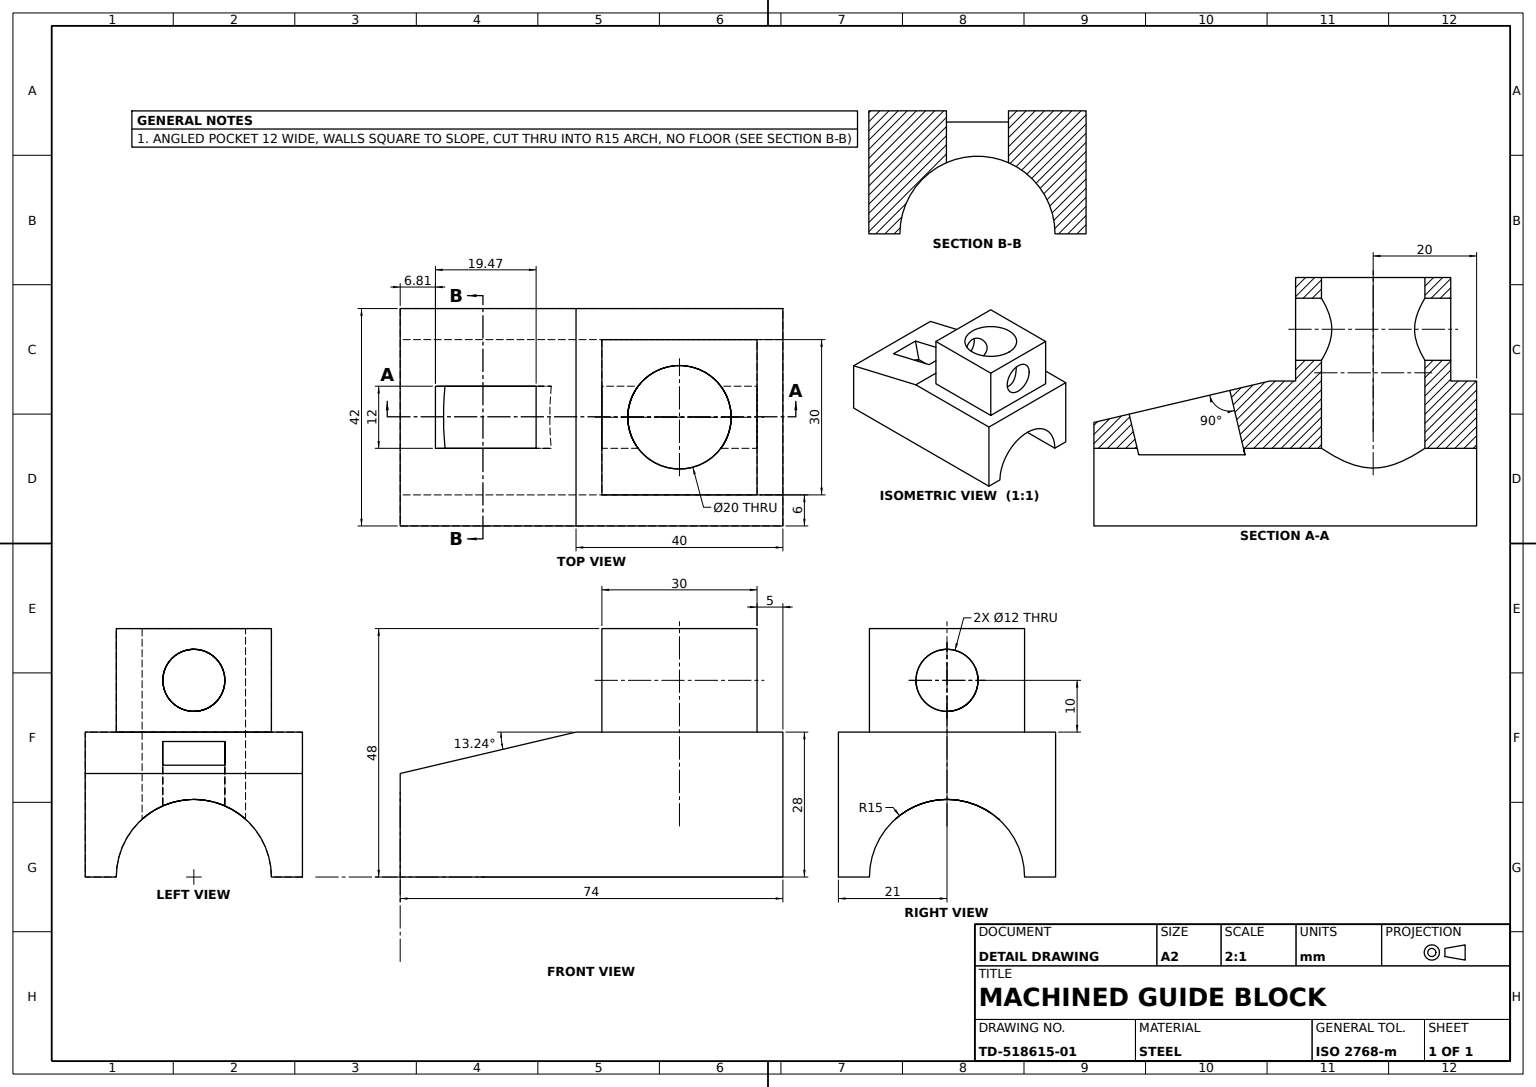
ISO-10303-21;
HEADER;
FILE_DESCRIPTION((''),'2;1');
FILE_NAME('','',(''),(''),'','','');
FILE_SCHEMA(('AUTOMOTIVE_DESIGN'));
ENDSEC;
DATA;
#1=APPLICATION_CONTEXT('');
#2=PRODUCT_CONTEXT('',#1,'mechanical');
#3=PRODUCT('','','',(#2));
#4=PRODUCT_DEFINITION_FORMATION('','',#3);
#5=PRODUCT_DEFINITION_CONTEXT('',#1,'design');
#6=PRODUCT_DEFINITION('','',#4,#5);
#7=PRODUCT_DEFINITION_SHAPE('','',#6);
#8=(LENGTH_UNIT()NAMED_UNIT(*)SI_UNIT(.MILLI.,.METRE.));
#9=(NAMED_UNIT(*)PLANE_ANGLE_UNIT()SI_UNIT($,.RADIAN.));
#10=(NAMED_UNIT(*)SI_UNIT($,.STERADIAN.)SOLID_ANGLE_UNIT());
#11=UNCERTAINTY_MEASURE_WITH_UNIT(LENGTH_MEASURE(1.E-05),#8,'distance_accuracy_value','');
#12=(GEOMETRIC_REPRESENTATION_CONTEXT(3)GLOBAL_UNCERTAINTY_ASSIGNED_CONTEXT((#11))GLOBAL_UNIT_ASSIGNED_CONTEXT((#8,#9,#10))REPRESENTATION_CONTEXT('',''));
#13=CARTESIAN_POINT('',(69.,28.,6.));
#14=VERTEX_POINT('',#13);
#15=CARTESIAN_POINT('',(39.,28.,6.));
#16=VERTEX_POINT('',#15);
#17=DIRECTION('',(-1.,0.,0.));
#18=VECTOR('',#17,1000.);
#19=LINE('',#15,#18);
#20=EDGE_CURVE('',#14,#16,#19,.T.);
#21=ORIENTED_EDGE('',*,*,#20,.T.);
#22=CARTESIAN_POINT('',(39.,48.,6.));
#23=VERTEX_POINT('',#22);
#24=DIRECTION('',(0.,-1.,0.));
#25=VECTOR('',#24,1000.);
#26=LINE('',#22,#25);
#27=EDGE_CURVE('',#23,#16,#26,.T.);
#28=ORIENTED_EDGE('',*,*,#27,.F.);
#29=CARTESIAN_POINT('',(69.,48.,6.));
#30=VERTEX_POINT('',#29);
#31=LINE('',#22,#18);
#32=EDGE_CURVE('',#30,#23,#31,.T.);
#33=ORIENTED_EDGE('',*,*,#32,.F.);
#34=LINE('',#29,#25);
#35=EDGE_CURVE('',#30,#14,#34,.T.);
#36=ORIENTED_EDGE('',*,*,#35,.T.);
#37=EDGE_LOOP('',(#21,#28,#33,#36));
#38=FACE_OUTER_BOUND('',#37,.T.);
#39=DIRECTION('',(0.,0.,1.));
#40=DIRECTION('',(1.,0.,0.));
#41=AXIS2_PLACEMENT_3D('',#22,#39,#40);
#42=PLANE('',#41);
#43=ADVANCED_FACE('',(#38),#42,.F.);
#44=CARTESIAN_POINT('',(8.662284,13.747727,27.));
#45=VERTEX_POINT('',#44);
#46=CARTESIAN_POINT('',(6.81392,21.603275,27.));
#47=VERTEX_POINT('',#46);
#48=CARTESIAN_POINT('',(15.154904,-13.845905,27.));
#49=DIRECTION('',(-0.229039334,0.973417168,0.));
#50=VECTOR('',#49,1000.);
#51=LINE('',#48,#50);
#52=EDGE_CURVE('',#45,#47,#51,.T.);
#53=ORIENTED_EDGE('',*,*,#52,.F.);
#54=CARTESIAN_POINT('',(8.662284,13.747727,15.));
#55=VERTEX_POINT('',#54);
#56=CARTESIAN_POINT('',(8.263626,15.442026,23.117874));
#57=CARTESIAN_POINT('',(8.263626,15.442026,18.882126));
#58=(BOUNDED_CURVE()B_SPLINE_CURVE(3,(#44,#56,#57,#54),.UNSPECIFIED.,.F.,.F.)B_SPLINE_CURVE_WITH_KNOTS((4,4),(5.871668461,6.694702153),.UNSPECIFIED.)CURVE()GEOMETRIC_REPRESENTATION_ITEM()RATIONAL_B_SPLINE_CURVE((1.,0.944343426,0.944343426,1.))REPRESENTATION_ITEM(''));
#59=EDGE_CURVE('',#45,#55,#58,.T.);
#60=ORIENTED_EDGE('',*,*,#59,.T.);
#61=CARTESIAN_POINT('',(6.81392,21.603275,15.));
#62=VERTEX_POINT('',#61);
#63=CARTESIAN_POINT('',(15.154904,-13.845905,15.));
#64=LINE('',#63,#50);
#65=EDGE_CURVE('',#55,#62,#64,.T.);
#66=ORIENTED_EDGE('',*,*,#65,.T.);
#67=CARTESIAN_POINT('',(6.81392,21.603275,21.));
#68=VECTOR('',#39,1000.);
#69=LINE('',#67,#68);
#70=EDGE_CURVE('',#62,#47,#69,.T.);
#71=ORIENTED_EDGE('',*,*,#70,.T.);
#72=EDGE_LOOP('',(#53,#60,#66,#71));
#73=FACE_OUTER_BOUND('',#72,.T.);
#74=CARTESIAN_POINT('',(15.154904,-13.845905,21.));
#75=DIRECTION('',(-0.973417168,-0.229039334,0.));
#76=DIRECTION('',(0.229039334,-0.973417168,0.));
#77=AXIS2_PLACEMENT_3D('',#74,#75,#76);
#78=PLANE('',#77);
#79=ADVANCED_FACE('',(#73),#78,.F.);
#80=CARTESIAN_POINT('',(44.,15.,21.));
#81=VERTEX_POINT('',#80);
#82=CARTESIAN_POINT('',(64.,15.,21.));
#83=VERTEX_POINT('',#82);
#84=CARTESIAN_POINT('',(44.,15.,20.315766));
#85=CARTESIAN_POINT('',(44.069456,14.953444,19.646642));
#86=CARTESIAN_POINT('',(44.338112,14.776396,18.336319));
#87=CARTESIAN_POINT('',(44.540827,14.643657,17.690301));
#88=CARTESIAN_POINT('',(45.054072,14.317485,16.483317));
#89=CARTESIAN_POINT('',(45.365864,14.123132,15.913734));
#90=CARTESIAN_POINT('',(46.093085,13.690648,14.843775));
#91=CARTESIAN_POINT('',(46.499373,13.457922,14.35618));
#92=CARTESIAN_POINT('',(47.39588,12.979625,13.464394));
#93=CARTESIAN_POINT('',(47.891028,12.7318,13.057623));
#94=CARTESIAN_POINT('',(48.941558,12.262423,12.350546));
#95=CARTESIAN_POINT('',(49.498495,12.039444,12.047121));
#96=CARTESIAN_POINT('',(50.390776,11.745112,11.668446));
#97=CARTESIAN_POINT('',(50.699259,11.653393,11.554638));
#98=CARTESIAN_POINT('',(51.33166,11.490287,11.356882));
#99=CARTESIAN_POINT('',(51.65257,11.419613,11.27373));
#100=CARTESIAN_POINT('',(52.304444,11.303629,11.139176));
#101=CARTESIAN_POINT('',(52.635408,11.258325,11.087771));
#102=CARTESIAN_POINT('',(53.308259,11.196708,11.018222));
#103=CARTESIAN_POINT('',(53.652096,11.180607,11.000299));
#104=CARTESIAN_POINT('',(54.669733,11.179816,10.999414));
#105=CARTESIAN_POINT('',(55.33834,11.241429,11.067135));
#106=CARTESIAN_POINT('',(56.327525,11.415429,11.26882));
#107=CARTESIAN_POINT('',(56.651266,11.486374,11.352241));
#108=CARTESIAN_POINT('',(57.280293,11.647657,11.547586));
#109=CARTESIAN_POINT('',(57.586917,11.738226,11.659782));
#110=CARTESIAN_POINT('',(58.18588,11.934889,11.912423));
#111=CARTESIAN_POINT('',(58.479453,12.0415,12.053601));
#112=CARTESIAN_POINT('',(59.045381,12.263283,12.360111));
#113=CARTESIAN_POINT('',(59.318063,12.37846,12.525395));
#114=CARTESIAN_POINT('',(59.844751,12.613707,12.879679));
#115=CARTESIAN_POINT('',(60.098751,12.733786,13.068682));
#116=CARTESIAN_POINT('',(60.589028,12.97574,13.471037));
#117=CARTESIAN_POINT('',(60.826316,13.098175,13.685453));
#118=CARTESIAN_POINT('',(61.502941,13.459144,14.358416));
#119=CARTESIAN_POINT('',(61.907554,13.691086,14.845407));
#120=CARTESIAN_POINT('',(62.4469,14.011753,15.637912));
#121=CARTESIAN_POINT('',(62.615307,14.114119,15.912494));
#122=CARTESIAN_POINT('',(62.928321,14.307332,16.484325));
#123=CARTESIAN_POINT('',(63.07303,14.398263,16.782352));
#124=CARTESIAN_POINT('',(63.459729,14.644004,17.691343));
#125=CARTESIAN_POINT('',(63.65875,14.774335,18.323429));
#126=CARTESIAN_POINT('',(63.862792,14.908791,19.315004));
#127=CARTESIAN_POINT('',(63.914681,14.943234,19.653364));
#128=CARTESIAN_POINT('',(63.982998,14.988649,20.326153));
#129=CARTESIAN_POINT('',(64.,15.,20.662901));
#130=B_SPLINE_CURVE_WITH_KNOTS('',3,(#80,#84,#85,#86,#87,#88,#89,#90,#91,#92,#93,#94,#95,#96,#97,#98,#99,#100,#101,#102,#103,#104,#105,#106,#107,#108,#109,#110,#111,#112,#113,#114,#115,#116,#117,#118,#119,#120,#121,#122,#123,#124,#125,#126,#127,#128,#129,#82),.UNSPECIFIED.,.F.,.F.,(4,2,2,2,2,2,2,2,2,2,2,2,2,2,2,2,2,2,2,2,2,2,2,4),(0.,0.002019983,0.004039966,0.006059949,0.008079932,0.010099915,0.012119898,0.013129889,0.014139881,0.015149872,0.016159864,0.018179847,0.019189838,0.02019983,0.021209821,0.022219812,0.023229804,0.024239795,0.026259778,0.02726977,0.028279761,0.030299744,0.031309736,0.032319727),.UNSPECIFIED.);
#131=EDGE_CURVE('',#81,#83,#130,.T.);
#132=ORIENTED_EDGE('',*,*,#131,.F.);
#133=CARTESIAN_POINT('',(64.,15.,21.336653));
#134=CARTESIAN_POINT('',(63.983044,14.98868,21.673657));
#135=CARTESIAN_POINT('',(63.914478,14.943099,22.348377));
#136=CARTESIAN_POINT('',(63.862521,14.908613,22.686291));
#137=CARTESIAN_POINT('',(63.659358,14.774736,23.673654));
#138=CARTESIAN_POINT('',(63.460738,14.64464,24.306492));
#139=CARTESIAN_POINT('',(63.071809,14.397489,25.220414));
#140=CARTESIAN_POINT('',(62.927942,14.3071,25.516335));
#141=CARTESIAN_POINT('',(62.616155,14.114641,26.085991));
#142=CARTESIAN_POINT('',(62.447797,14.012288,26.360755));
#143=CARTESIAN_POINT('',(61.90617,13.69026,27.156655));
#144=CARTESIAN_POINT('',(61.492918,13.4536,27.652569));
#145=CARTESIAN_POINT('',(60.594478,12.974694,28.544094));
#146=CARTESIAN_POINT('',(60.107726,12.731094,28.943623));
#147=CARTESIAN_POINT('',(59.31506,12.377155,29.476526));
#148=CARTESIAN_POINT('',(59.039253,12.260777,29.643428));
#149=CARTESIAN_POINT('',(58.474857,12.039806,29.948664));
#150=CARTESIAN_POINT('',(58.185318,11.934736,30.087761));
#151=CARTESIAN_POINT('',(57.590293,11.739303,30.338847));
#152=CARTESIAN_POINT('',(57.284813,11.648933,30.450844));
#153=CARTESIAN_POINT('',(56.655932,11.487455,30.646474));
#154=CARTESIAN_POINT('',(56.330246,11.416025,30.730479));
#155=CARTESIAN_POINT('',(55.345423,11.242442,30.931711));
#156=CARTESIAN_POINT('',(54.676284,11.179925,31.000464));
#157=CARTESIAN_POINT('',(53.651615,11.180551,30.999764));
#158=CARTESIAN_POINT('',(53.310132,11.196628,30.981866));
#159=CARTESIAN_POINT('',(52.639673,11.257844,30.912774));
#160=CARTESIAN_POINT('',(52.30873,11.302959,30.861593));
#161=CARTESIAN_POINT('',(51.654892,11.419108,30.726864));
#162=CARTESIAN_POINT('',(51.330007,11.490688,30.642637));
#163=CARTESIAN_POINT('',(50.698906,11.653509,30.445215));
#164=CARTESIAN_POINT('',(50.393107,11.7444,30.332447));
#165=CARTESIAN_POINT('',(49.501422,12.038365,29.954313));
#166=CARTESIAN_POINT('',(48.94037,12.262732,29.649261));
#167=CARTESIAN_POINT('',(47.8791,12.737353,28.933735));
#168=CARTESIAN_POINT('',(47.39227,12.98147,28.532433));
#169=CARTESIAN_POINT('',(46.720293,13.3401,27.863365));
#170=CARTESIAN_POINT('',(46.506134,13.458444,27.629057));
#171=CARTESIAN_POINT('',(46.09759,13.690134,27.136314));
#172=CARTESIAN_POINT('',(45.903795,13.803175,26.878281));
#173=CARTESIAN_POINT('',(45.364101,14.124275,26.082531));
#174=CARTESIAN_POINT('',(45.055173,14.316803,25.51853));
#175=CARTESIAN_POINT('',(44.671193,14.560799,24.616644));
#176=CARTESIAN_POINT('',(44.556546,14.634651,24.306638));
#177=CARTESIAN_POINT('',(44.356066,14.764811,23.665935));
#178=CARTESIAN_POINT('',(44.27196,14.819993,23.340409));
#179=CARTESIAN_POINT('',(44.069686,14.953289,22.355722));
#180=CARTESIAN_POINT('',(44.,15.,21.68333));
#181=B_SPLINE_CURVE_WITH_KNOTS('',3,(#82,#133,#134,#135,#136,#137,#138,#139,#140,#141,#142,#143,#144,#145,#146,#147,#148,#149,#150,#151,#152,#153,#154,#155,#156,#157,#158,#159,#160,#161,#162,#163,#164,#165,#166,#167,#168,#169,#170,#171,#172,#173,#174,#175,#176,#177,#178,#179,#180,#80),.UNSPECIFIED.,.F.,.F.,(4,2,2,2,2,2,2,2,2,2,2,2,2,2,2,2,2,2,2,2,2,2,2,2,4),(0.032319727,0.033328384,0.034337041,0.036354356,0.037363013,0.03837167,0.040388984,0.042406298,0.043414955,0.044423612,0.04543227,0.046440927,0.048458241,0.049466898,0.050475555,0.051484212,0.052492869,0.054510184,0.056527498,0.057536155,0.058544812,0.060562126,0.061570783,0.06257944,0.064596755),.UNSPECIFIED.);
#182=EDGE_CURVE('',#83,#81,#181,.T.);
#183=ORIENTED_EDGE('',*,*,#182,.F.);
#184=EDGE_LOOP('',(#132,#183));
#185=FACE_BOUND('',#184,.T.);
#186=CARTESIAN_POINT('',(0.,0.,6.));
#187=VERTEX_POINT('',#186);
#188=CARTESIAN_POINT('',(0.,0.,36.));
#189=VERTEX_POINT('',#188);
#190=CARTESIAN_POINT('',(0.,0.,21.));
#191=DIRECTION('',(0.,1.,0.));
#192=AXIS2_PLACEMENT_3D('',#190,#40,#191);
#193=CIRCLE('',#192,15.);
#194=EDGE_CURVE('',#187,#189,#193,.T.);
#195=ORIENTED_EDGE('',*,*,#194,.F.);
#196=CARTESIAN_POINT('',(74.,0.,6.));
#197=VERTEX_POINT('',#196);
#198=CARTESIAN_POINT('',(164.616747,0.,6.));
#199=LINE('',#198,#18);
#200=EDGE_CURVE('',#197,#187,#199,.T.);
#201=ORIENTED_EDGE('',*,*,#200,.F.);
#202=CARTESIAN_POINT('',(74.,0.,36.));
#203=VERTEX_POINT('',#202);
#204=CARTESIAN_POINT('',(74.,0.,21.));
#205=AXIS2_PLACEMENT_3D('',#204,#17,#39);
#206=CIRCLE('',#205,15.);
#207=EDGE_CURVE('',#203,#197,#206,.T.);
#208=ORIENTED_EDGE('',*,*,#207,.F.);
#209=CARTESIAN_POINT('',(164.616747,0.,36.));
#210=LINE('',#209,#18);
#211=EDGE_CURVE('',#203,#189,#210,.T.);
#212=ORIENTED_EDGE('',*,*,#211,.T.);
#213=EDGE_LOOP('',(#195,#201,#208,#212));
#214=FACE_OUTER_BOUND('',#213,.T.);
#215=CARTESIAN_POINT('',(29.20846,13.747727,15.));
#216=VERTEX_POINT('',#215);
#217=CARTESIAN_POINT('',(29.20846,13.747727,27.));
#218=VERTEX_POINT('',#217);
#219=CARTESIAN_POINT('',(28.809801,15.442026,18.882126));
#220=CARTESIAN_POINT('',(28.809801,15.442026,23.117874));
#221=(BOUNDED_CURVE()B_SPLINE_CURVE(3,(#215,#219,#220,#217),.UNSPECIFIED.,.F.,.F.)B_SPLINE_CURVE_WITH_KNOTS((4,4),(5.871668461,6.694702153),.UNSPECIFIED.)CURVE()GEOMETRIC_REPRESENTATION_ITEM()RATIONAL_B_SPLINE_CURVE((1.,0.944343426,0.944343426,1.))REPRESENTATION_ITEM(''));
#222=EDGE_CURVE('',#216,#218,#221,.T.);
#223=ORIENTED_EDGE('',*,*,#222,.F.);
#224=CARTESIAN_POINT('',(164.616747,13.747727,15.));
#225=VECTOR('',#40,1000.);
#226=LINE('',#224,#225);
#227=EDGE_CURVE('',#55,#216,#226,.T.);
#228=ORIENTED_EDGE('',*,*,#227,.F.);
#229=ORIENTED_EDGE('',*,*,#59,.F.);
#230=CARTESIAN_POINT('',(164.616747,13.747727,27.));
#231=LINE('',#230,#18);
#232=EDGE_CURVE('',#218,#45,#231,.T.);
#233=ORIENTED_EDGE('',*,*,#232,.F.);
#234=EDGE_LOOP('',(#223,#228,#229,#233));
#235=FACE_BOUND('',#234,.T.);
#236=CARTESIAN_POINT('',(164.616747,0.,21.));
#237=AXIS2_PLACEMENT_3D('',#236,#17,#24);
#238=CYLINDRICAL_SURFACE('',#237,15.);
#239=ADVANCED_FACE('',(#185,#214,#235),#238,.F.);
#240=CARTESIAN_POINT('',(0.,0.,42.));
#241=VERTEX_POINT('',#240);
#242=DIRECTION('',(0.,0.,-1.));
#243=VECTOR('',#242,1000.);
#244=LINE('',#240,#243);
#245=EDGE_CURVE('',#241,#189,#244,.T.);
#246=ORIENTED_EDGE('',*,*,#245,.F.);
#247=CARTESIAN_POINT('',(0.,20.,42.));
#248=VERTEX_POINT('',#247);
#249=LINE('',#247,#25);
#250=EDGE_CURVE('',#248,#241,#249,.T.);
#251=ORIENTED_EDGE('',*,*,#250,.F.);
#252=CARTESIAN_POINT('',(0.,20.,0.));
#253=VERTEX_POINT('',#252);
#254=LINE('',#247,#243);
#255=EDGE_CURVE('',#248,#253,#254,.T.);
#256=ORIENTED_EDGE('',*,*,#255,.T.);
#257=CARTESIAN_POINT('',(0.,0.,0.));
#258=VERTEX_POINT('',#257);
#259=LINE('',#252,#25);
#260=EDGE_CURVE('',#253,#258,#259,.T.);
#261=ORIENTED_EDGE('',*,*,#260,.T.);
#262=EDGE_CURVE('',#187,#258,#244,.T.);
#263=ORIENTED_EDGE('',*,*,#262,.F.);
#264=ORIENTED_EDGE('',*,*,#194,.T.);
#265=EDGE_LOOP('',(#246,#251,#256,#261,#263,#264));
#266=FACE_OUTER_BOUND('',#265,.T.);
#267=AXIS2_PLACEMENT_3D('',#247,#40,#191);
#268=PLANE('',#267);
#269=ADVANCED_FACE('',(#266),#268,.F.);
#270=CARTESIAN_POINT('',(26.282264,26.184062,15.));
#271=VERTEX_POINT('',#270);
#272=CARTESIAN_POINT('',(34.623247,-9.265118,15.));
#273=LINE('',#272,#50);
#274=EDGE_CURVE('',#216,#271,#273,.T.);
#275=ORIENTED_EDGE('',*,*,#274,.F.);
#276=ORIENTED_EDGE('',*,*,#222,.T.);
#277=CARTESIAN_POINT('',(26.282264,26.184062,27.));
#278=VERTEX_POINT('',#277);
#279=CARTESIAN_POINT('',(34.623247,-9.265118,27.));
#280=LINE('',#279,#50);
#281=EDGE_CURVE('',#218,#278,#280,.T.);
#282=ORIENTED_EDGE('',*,*,#281,.T.);
#283=LINE('',#270,#243);
#284=EDGE_CURVE('',#278,#271,#283,.T.);
#285=ORIENTED_EDGE('',*,*,#284,.T.);
#286=EDGE_LOOP('',(#275,#276,#282,#285));
#287=FACE_OUTER_BOUND('',#286,.T.);
#288=DIRECTION('',(0.973417168,0.229039334,0.));
#289=AXIS2_PLACEMENT_3D('',#272,#288,#49);
#290=PLANE('',#289);
#291=ADVANCED_FACE('',(#287),#290,.F.);
#292=ORIENTED_EDGE('',*,*,#200,.T.);
#293=ORIENTED_EDGE('',*,*,#262,.T.);
#294=CARTESIAN_POINT('',(74.,0.,0.));
#295=VERTEX_POINT('',#294);
#296=LINE('',#257,#225);
#297=EDGE_CURVE('',#258,#295,#296,.T.);
#298=ORIENTED_EDGE('',*,*,#297,.T.);
#299=CARTESIAN_POINT('',(74.,0.,42.));
#300=LINE('',#299,#243);
#301=EDGE_CURVE('',#197,#295,#300,.T.);
#302=ORIENTED_EDGE('',*,*,#301,.F.);
#303=EDGE_LOOP('',(#292,#293,#298,#302));
#304=FACE_OUTER_BOUND('',#303,.T.);
#305=AXIS2_PLACEMENT_3D('',#240,#191,#39);
#306=PLANE('',#305);
#307=ADVANCED_FACE('',(#304),#306,.F.);
#308=CARTESIAN_POINT('',(69.,28.,36.));
#309=VERTEX_POINT('',#308);
#310=LINE('',#13,#243);
#311=EDGE_CURVE('',#309,#14,#310,.T.);
#312=ORIENTED_EDGE('',*,*,#311,.F.);
#313=CARTESIAN_POINT('',(39.,28.,36.));
#314=VERTEX_POINT('',#313);
#315=LINE('',#313,#225);
#316=EDGE_CURVE('',#314,#309,#315,.T.);
#317=ORIENTED_EDGE('',*,*,#316,.F.);
#318=LINE('',#15,#68);
#319=EDGE_CURVE('',#16,#314,#318,.T.);
#320=ORIENTED_EDGE('',*,*,#319,.F.);
#321=ORIENTED_EDGE('',*,*,#20,.F.);
#322=EDGE_LOOP('',(#312,#317,#320,#321));
#323=FACE_BOUND('',#322,.T.);
#324=CARTESIAN_POINT('',(34.,28.,42.));
#325=VERTEX_POINT('',#324);
#326=CARTESIAN_POINT('',(34.,28.,0.));
#327=VERTEX_POINT('',#326);
#328=LINE('',#324,#243);
#329=EDGE_CURVE('',#325,#327,#328,.T.);
#330=ORIENTED_EDGE('',*,*,#329,.F.);
#331=CARTESIAN_POINT('',(74.,28.,42.));
#332=VERTEX_POINT('',#331);
#333=LINE('',#331,#18);
#334=EDGE_CURVE('',#332,#325,#333,.T.);
#335=ORIENTED_EDGE('',*,*,#334,.F.);
#336=CARTESIAN_POINT('',(74.,28.,0.));
#337=VERTEX_POINT('',#336);
#338=LINE('',#331,#243);
#339=EDGE_CURVE('',#332,#337,#338,.T.);
#340=ORIENTED_EDGE('',*,*,#339,.T.);
#341=LINE('',#336,#18);
#342=EDGE_CURVE('',#337,#327,#341,.T.);
#343=ORIENTED_EDGE('',*,*,#342,.T.);
#344=EDGE_LOOP('',(#330,#335,#340,#343));
#345=FACE_OUTER_BOUND('',#344,.T.);
#346=AXIS2_PLACEMENT_3D('',#331,#24,#40);
#347=PLANE('',#346);
#348=ADVANCED_FACE('',(#323,#345),#347,.F.);
#349=CARTESIAN_POINT('',(69.,38.,15.));
#350=VERTEX_POINT('',#349);
#351=CARTESIAN_POINT('',(69.,38.,27.));
#352=VERTEX_POINT('',#351);
#353=CARTESIAN_POINT('',(69.,38.,21.));
#354=AXIS2_PLACEMENT_3D('',#353,#17,#24);
#355=CIRCLE('',#354,6.);
#356=EDGE_CURVE('',#350,#352,#355,.T.);
#357=ORIENTED_EDGE('',*,*,#356,.F.);
#358=CARTESIAN_POINT('',(62.,38.,15.));
#359=VERTEX_POINT('',#358);
#360=CARTESIAN_POINT('',(74.,38.,15.));
#361=LINE('',#360,#18);
#362=EDGE_CURVE('',#350,#359,#361,.T.);
#363=ORIENTED_EDGE('',*,*,#362,.T.);
#364=CARTESIAN_POINT('',(64.,32.,21.));
#365=VERTEX_POINT('',#364);
#366=CARTESIAN_POINT('',(64.,32.,20.797821));
#367=CARTESIAN_POINT('',(63.993753,32.010394,20.593631));
#368=CARTESIAN_POINT('',(63.969415,32.051092,20.193152));
#369=CARTESIAN_POINT('',(63.951355,32.081342,19.995381));
#370=CARTESIAN_POINT('',(63.904121,32.161109,19.604607));
#371=CARTESIAN_POINT('',(63.874944,32.210627,19.411603));
#372=CARTESIAN_POINT('',(63.806013,32.329003,19.030319));
#373=CARTESIAN_POINT('',(63.766263,32.397869,18.842476));
#374=CARTESIAN_POINT('',(63.635373,32.628186,18.298376));
#375=CARTESIAN_POINT('',(63.531871,32.814358,17.956932));
#376=CARTESIAN_POINT('',(63.301834,33.250428,17.31317));
#377=CARTESIAN_POINT('',(63.177176,33.496923,17.016551));
#378=CARTESIAN_POINT('',(62.987483,33.902545,16.612831));
#379=CARTESIAN_POINT('',(62.92364,34.044086,16.484748));
#380=CARTESIAN_POINT('',(62.796288,34.340413,16.24141));
#381=CARTESIAN_POINT('',(62.732524,34.495907,16.125753));
#382=CARTESIAN_POINT('',(62.547842,34.974718,15.804282));
#383=CARTESIAN_POINT('',(62.432517,35.312013,15.621767));
#384=CARTESIAN_POINT('',(62.282471,35.848533,15.39564));
#385=CARTESIAN_POINT('',(62.236305,36.032511,15.328277));
#386=CARTESIAN_POINT('',(62.153993,36.411952,15.210565));
#387=CARTESIAN_POINT('',(62.118165,36.606454,15.160667));
#388=CARTESIAN_POINT('',(62.031323,37.192788,15.041179));
#389=CARTESIAN_POINT('',(62.,37.592241,15.));
#390=B_SPLINE_CURVE_WITH_KNOTS('',3,(#364,#366,#367,#368,#369,#370,#371,#372,#373,#374,#375,#376,#377,#378,#379,#380,#381,#382,#383,#384,#385,#386,#387,#388,#389,#358),.UNSPECIFIED.,.F.,.F.,(4,2,2,2,2,2,2,2,2,2,2,2,4),(0.009631544,0.01023216,0.010832776,0.011433391,0.012034007,0.013235238,0.01443647,0.015037085,0.015637701,0.016838933,0.017439548,0.018040164,0.019241395),.UNSPECIFIED.);
#391=EDGE_CURVE('',#365,#359,#390,.T.);
#392=ORIENTED_EDGE('',*,*,#391,.F.);
#393=CARTESIAN_POINT('',(62.,38.,27.));
#394=VERTEX_POINT('',#393);
#395=CARTESIAN_POINT('',(62.,37.591768,27.));
#396=CARTESIAN_POINT('',(62.031328,37.193184,26.958808));
#397=CARTESIAN_POINT('',(62.146708,36.413314,26.800067));
#398=CARTESIAN_POINT('',(62.231957,36.029098,26.680494));
#399=CARTESIAN_POINT('',(62.433243,35.309475,26.377132));
#400=CARTESIAN_POINT('',(62.54964,34.969458,26.192873));
#401=CARTESIAN_POINT('',(62.798002,34.326762,25.759983));
#402=CARTESIAN_POINT('',(62.926719,34.032198,25.516923));
#403=CARTESIAN_POINT('',(63.11667,33.626449,25.112002));
#404=CARTESIAN_POINT('',(63.179494,33.497283,24.970247));
#405=CARTESIAN_POINT('',(63.302673,33.251204,24.672364));
#406=CARTESIAN_POINT('',(63.362926,33.134529,24.516325));
#407=CARTESIAN_POINT('',(63.534158,32.810213,24.035708));
#408=CARTESIAN_POINT('',(63.636973,32.625336,23.695716));
#409=CARTESIAN_POINT('',(63.81049,32.320081,22.972921));
#410=CARTESIAN_POINT('',(63.881397,32.199475,22.585282));
#411=CARTESIAN_POINT('',(63.975468,32.040633,21.803219));
#412=CARTESIAN_POINT('',(64.,32.,21.40527));
#413=B_SPLINE_CURVE_WITH_KNOTS('',3,(#393,#395,#396,#397,#398,#399,#400,#401,#402,#403,#404,#405,#406,#407,#408,#409,#410,#411,#412,#364),.UNSPECIFIED.,.F.,.F.,(4,2,2,2,2,2,2,2,2,4),(0.,0.001203943,0.002407886,0.003611829,0.004815772,0.005417744,0.006019715,0.007223658,0.008427601,0.009631544),.UNSPECIFIED.);
#414=EDGE_CURVE('',#394,#365,#413,.T.);
#415=ORIENTED_EDGE('',*,*,#414,.F.);
#416=CARTESIAN_POINT('',(74.,38.,27.));
#417=LINE('',#416,#18);
#418=EDGE_CURVE('',#352,#394,#417,.T.);
#419=ORIENTED_EDGE('',*,*,#418,.F.);
#420=EDGE_LOOP('',(#357,#363,#392,#415,#419));
#421=FACE_OUTER_BOUND('',#420,.T.);
#422=CARTESIAN_POINT('',(74.,38.,21.));
#423=AXIS2_PLACEMENT_3D('',#422,#17,#39);
#424=CYLINDRICAL_SURFACE('',#423,6.);
#425=ADVANCED_FACE('',(#421),#424,.F.);
#426=CARTESIAN_POINT('',(46.,38.,27.));
#427=VERTEX_POINT('',#426);
#428=CARTESIAN_POINT('',(39.,38.,27.));
#429=VERTEX_POINT('',#428);
#430=EDGE_CURVE('',#427,#429,#417,.T.);
#431=ORIENTED_EDGE('',*,*,#430,.F.);
#432=CARTESIAN_POINT('',(44.,32.,21.));
#433=VERTEX_POINT('',#432);
#434=CARTESIAN_POINT('',(44.,32.,21.407499));
#435=CARTESIAN_POINT('',(44.024793,32.041068,21.806407));
#436=CARTESIAN_POINT('',(44.119086,32.200295,22.588264));
#437=CARTESIAN_POINT('',(44.189825,32.320615,22.974634));
#438=CARTESIAN_POINT('',(44.363887,32.626868,23.698897));
#439=CARTESIAN_POINT('',(44.467296,32.812819,24.040544));
#440=CARTESIAN_POINT('',(44.697713,33.249532,24.685758));
#441=CARTESIAN_POINT('',(44.821914,33.495068,24.981375));
#442=CARTESIAN_POINT('',(45.011717,33.900791,25.385536));
#443=CARTESIAN_POINT('',(45.075643,34.042462,25.513844));
#444=CARTESIAN_POINT('',(45.203249,34.339291,25.757742));
#445=CARTESIAN_POINT('',(45.266961,34.494638,25.873322));
#446=CARTESIAN_POINT('',(45.451379,34.97257,26.194421));
#447=CARTESIAN_POINT('',(45.566775,35.309727,26.377137));
#448=CARTESIAN_POINT('',(45.767285,36.026203,26.679375));
#449=CARTESIAN_POINT('',(45.852727,36.410305,26.799279));
#450=CARTESIAN_POINT('',(45.939547,36.995927,26.918744));
#451=CARTESIAN_POINT('',(45.961914,37.193427,26.948934));
#452=CARTESIAN_POINT('',(45.992147,37.593247,26.989568));
#453=CARTESIAN_POINT('',(46.,37.796773,27.));
#454=B_SPLINE_CURVE_WITH_KNOTS('',3,(#432,#434,#435,#436,#437,#438,#439,#440,#441,#442,#443,#444,#445,#446,#447,#448,#449,#450,#451,#452,#453,#426),.UNSPECIFIED.,.F.,.F.,(4,2,2,2,2,2,2,2,2,2,4),(0.,0.001203351,0.002406702,0.003610054,0.004813405,0.00541508,0.006016756,0.007220107,0.008423459,0.009025134,0.00962681),.UNSPECIFIED.);
#455=EDGE_CURVE('',#433,#427,#454,.T.);
#456=ORIENTED_EDGE('',*,*,#455,.F.);
#457=CARTESIAN_POINT('',(46.,38.,15.));
#458=VERTEX_POINT('',#457);
#459=CARTESIAN_POINT('',(46.,37.597109,15.));
#460=CARTESIAN_POINT('',(45.969424,37.198811,15.040164));
#461=CARTESIAN_POINT('',(45.853035,36.411041,15.200279));
#462=CARTESIAN_POINT('',(45.768824,36.032314,15.318377));
#463=CARTESIAN_POINT('',(45.567625,35.312161,15.621511));
#464=CARTESIAN_POINT('',(45.449548,34.967446,15.808587));
#465=CARTESIAN_POINT('',(45.203681,34.331025,16.237042));
#466=CARTESIAN_POINT('',(45.074985,34.035885,16.479513));
#467=CARTESIAN_POINT('',(44.819146,33.489301,17.024751));
#468=CARTESIAN_POINT('',(44.695693,33.245677,17.319768));
#469=CARTESIAN_POINT('',(44.525252,32.922676,17.797234));
#470=CARTESIAN_POINT('',(44.470881,32.822147,17.96226));
#471=CARTESIAN_POINT('',(44.368373,32.635833,18.304868));
#472=CARTESIAN_POINT('',(44.319959,32.54957,18.483684));
#473=CARTESIAN_POINT('',(44.188886,32.318983,19.029678));
#474=CARTESIAN_POINT('',(44.120037,32.201914,19.406156));
#475=CARTESIAN_POINT('',(44.049147,32.082187,19.99053));
#476=CARTESIAN_POINT('',(44.030925,32.051662,20.188618));
#477=CARTESIAN_POINT('',(44.006292,32.010471,20.591827));
#478=CARTESIAN_POINT('',(44.,32.,20.796725));
#479=B_SPLINE_CURVE_WITH_KNOTS('',3,(#457,#459,#460,#461,#462,#463,#464,#465,#466,#467,#468,#469,#470,#471,#472,#473,#474,#475,#476,#477,#478,#432),.UNSPECIFIED.,.F.,.F.,(4,2,2,2,2,2,2,2,2,2,4),(0.028856443,0.030056993,0.031257543,0.032458093,0.033658643,0.034859192,0.035459467,0.036059742,0.037260292,0.037860567,0.038460842),.UNSPECIFIED.);
#480=EDGE_CURVE('',#458,#433,#479,.T.);
#481=ORIENTED_EDGE('',*,*,#480,.F.);
#482=CARTESIAN_POINT('',(39.,38.,15.));
#483=VERTEX_POINT('',#482);
#484=EDGE_CURVE('',#458,#483,#361,.T.);
#485=ORIENTED_EDGE('',*,*,#484,.T.);
#486=CARTESIAN_POINT('',(39.,38.,21.));
#487=AXIS2_PLACEMENT_3D('',#486,#17,#39);
#488=CIRCLE('',#487,6.);
#489=EDGE_CURVE('',#483,#429,#488,.T.);
#490=ORIENTED_EDGE('',*,*,#489,.T.);
#491=EDGE_LOOP('',(#431,#456,#481,#485,#490));
#492=FACE_OUTER_BOUND('',#491,.T.);
#493=ADVANCED_FACE('',(#492),#424,.F.);
#494=VERTEX_POINT('',#299);
#495=EDGE_CURVE('',#494,#203,#300,.T.);
#496=ORIENTED_EDGE('',*,*,#495,.T.);
#497=ORIENTED_EDGE('',*,*,#207,.T.);
#498=ORIENTED_EDGE('',*,*,#301,.T.);
#499=VECTOR('',#191,1000.);
#500=LINE('',#294,#499);
#501=EDGE_CURVE('',#295,#337,#500,.T.);
#502=ORIENTED_EDGE('',*,*,#501,.T.);
#503=ORIENTED_EDGE('',*,*,#339,.F.);
#504=LINE('',#299,#499);
#505=EDGE_CURVE('',#494,#332,#504,.T.);
#506=ORIENTED_EDGE('',*,*,#505,.F.);
#507=EDGE_LOOP('',(#496,#497,#498,#502,#503,#506));
#508=FACE_OUTER_BOUND('',#507,.T.);
#509=AXIS2_PLACEMENT_3D('',#299,#17,#39);
#510=PLANE('',#509);
#511=ADVANCED_FACE('',(#508),#510,.F.);
#512=VECTOR('',#75,1000.);
#513=LINE('',#61,#512);
#514=EDGE_CURVE('',#271,#62,#513,.T.);
#515=ORIENTED_EDGE('',*,*,#514,.F.);
#516=ORIENTED_EDGE('',*,*,#284,.F.);
#517=VECTOR('',#288,1000.);
#518=LINE('',#277,#517);
#519=EDGE_CURVE('',#47,#278,#518,.T.);
#520=ORIENTED_EDGE('',*,*,#519,.F.);
#521=ORIENTED_EDGE('',*,*,#70,.F.);
#522=EDGE_LOOP('',(#515,#516,#520,#521));
#523=FACE_BOUND('',#522,.T.);
#524=LINE('',#326,#512);
#525=EDGE_CURVE('',#327,#253,#524,.T.);
#526=ORIENTED_EDGE('',*,*,#525,.T.);
#527=ORIENTED_EDGE('',*,*,#255,.F.);
#528=LINE('',#324,#512);
#529=EDGE_CURVE('',#325,#248,#528,.T.);
#530=ORIENTED_EDGE('',*,*,#529,.F.);
#531=ORIENTED_EDGE('',*,*,#329,.T.);
#532=EDGE_LOOP('',(#526,#527,#530,#531));
#533=FACE_OUTER_BOUND('',#532,.T.);
#534=AXIS2_PLACEMENT_3D('',#324,#76,#288);
#535=PLANE('',#534);
#536=ADVANCED_FACE('',(#523,#533),#535,.F.);
#537=ORIENTED_EDGE('',*,*,#362,.F.);
#538=EDGE_CURVE('',#352,#350,#355,.T.);
#539=ORIENTED_EDGE('',*,*,#538,.F.);
#540=ORIENTED_EDGE('',*,*,#418,.T.);
#541=CARTESIAN_POINT('',(64.,44.,21.));
#542=VERTEX_POINT('',#541);
#543=CARTESIAN_POINT('',(64.,44.,21.406914));
#544=CARTESIAN_POINT('',(63.975272,43.959042,21.806058));
#545=CARTESIAN_POINT('',(63.880713,43.799364,22.589747));
#546=CARTESIAN_POINT('',(63.809869,43.678858,22.976167));
#547=CARTESIAN_POINT('',(63.635663,43.372328,23.70051));
#548=CARTESIAN_POINT('',(63.5313,43.184602,24.044882));
#549=CARTESIAN_POINT('',(63.300972,42.747894,24.689026));
#550=CARTESIAN_POINT('',(63.177122,42.503003,24.983631));
#551=CARTESIAN_POINT('',(62.923505,41.960607,25.523266));
#552=CARTESIAN_POINT('',(62.792722,41.660341,25.769549));
#553=CARTESIAN_POINT('',(62.547483,41.024172,26.196256));
#554=CARTESIAN_POINT('',(62.431988,40.686631,26.379092));
#555=CARTESIAN_POINT('',(62.281153,40.146484,26.606314));
#556=CARTESIAN_POINT('',(62.234376,39.959382,26.674517));
#557=CARTESIAN_POINT('',(62.152522,39.580455,26.791501));
#558=CARTESIAN_POINT('',(62.117363,39.388689,26.840444));
#559=CARTESIAN_POINT('',(62.031348,38.806249,26.958771));
#560=CARTESIAN_POINT('',(62.,38.406877,27.));
#561=B_SPLINE_CURVE_WITH_KNOTS('',3,(#541,#543,#544,#545,#546,#547,#548,#549,#550,#551,#552,#553,#554,#555,#556,#557,#558,#559,#560,#393),.UNSPECIFIED.,.F.,.F.,(4,2,2,2,2,2,2,2,2,4),(0.028848506,0.030048453,0.031248401,0.032448349,0.033648296,0.034848244,0.036048192,0.036648166,0.037248139,0.038448087),.UNSPECIFIED.);
#562=EDGE_CURVE('',#542,#394,#561,.T.);
#563=ORIENTED_EDGE('',*,*,#562,.F.);
#564=CARTESIAN_POINT('',(62.,38.407643,15.));
#565=CARTESIAN_POINT('',(62.031251,38.806511,15.041083));
#566=CARTESIAN_POINT('',(62.11805,39.392873,15.160506));
#567=CARTESIAN_POINT('',(62.153861,39.587379,15.210379));
#568=CARTESIAN_POINT('',(62.236175,39.966954,15.328089));
#569=CARTESIAN_POINT('',(62.282464,40.151513,15.39562));
#570=CARTESIAN_POINT('',(62.38308,40.51114,15.547271));
#571=CARTESIAN_POINT('',(62.43741,40.686206,15.631393));
#572=CARTESIAN_POINT('',(62.552164,41.027428,15.816148));
#573=CARTESIAN_POINT('',(62.612817,41.194105,15.917207));
#574=CARTESIAN_POINT('',(62.798041,41.673183,16.240159));
#575=CARTESIAN_POINT('',(62.926533,41.967415,16.48266));
#576=CARTESIAN_POINT('',(63.180405,42.509683,17.023883));
#577=CARTESIAN_POINT('',(63.30609,42.757807,17.32423));
#578=CARTESIAN_POINT('',(63.533363,43.188296,17.961976));
#579=CARTESIAN_POINT('',(63.636376,43.373611,18.301843));
#580=CARTESIAN_POINT('',(63.767306,43.60395,18.847168));
#581=CARTESIAN_POINT('',(63.807113,43.672896,19.035867));
#582=CARTESIAN_POINT('',(63.875625,43.790531,19.415916));
#583=CARTESIAN_POINT('',(63.904622,43.83974,19.608269));
#584=CARTESIAN_POINT('',(63.975049,43.958664,20.19238));
#585=CARTESIAN_POINT('',(64.,44.,20.592767));
#586=B_SPLINE_CURVE_WITH_KNOTS('',3,(#358,#564,#565,#566,#567,#568,#569,#570,#571,#572,#573,#574,#575,#576,#577,#578,#579,#580,#581,#582,#583,#584,#585,#541),.UNSPECIFIED.,.F.,.F.,(4,2,2,2,2,2,2,2,2,2,2,4),(0.019241395,0.020442284,0.021042729,0.021643173,0.022243617,0.022844062,0.02404495,0.025245839,0.026446728,0.027047172,0.027647617,0.028848506),.UNSPECIFIED.);
#587=EDGE_CURVE('',#359,#542,#586,.T.);
#588=ORIENTED_EDGE('',*,*,#587,.F.);
#589=EDGE_LOOP('',(#537,#539,#540,#563,#588));
#590=FACE_OUTER_BOUND('',#589,.T.);
#591=ADVANCED_FACE('',(#590),#424,.F.);
#592=ORIENTED_EDGE('',*,*,#182,.T.);
#593=CARTESIAN_POINT('',(44.,0.,21.));
#594=LINE('',#593,#499);
#595=EDGE_CURVE('',#81,#433,#594,.T.);
#596=ORIENTED_EDGE('',*,*,#595,.T.);
#597=ORIENTED_EDGE('',*,*,#455,.T.);
#598=CARTESIAN_POINT('',(44.,44.,21.));
#599=VERTEX_POINT('',#598);
#600=CARTESIAN_POINT('',(46.,38.406283,27.));
#601=CARTESIAN_POINT('',(45.968942,38.804847,26.959179));
#602=CARTESIAN_POINT('',(45.8821,39.392041,26.839702));
#603=CARTESIAN_POINT('',(45.846194,39.587061,26.789696));
#604=CARTESIAN_POINT('',(45.764049,39.965983,26.672235));
#605=CARTESIAN_POINT('',(45.717824,40.150404,26.604805));
#606=CARTESIAN_POINT('',(45.566959,40.689871,26.377445));
#607=CARTESIAN_POINT('',(45.449031,41.034077,26.190601));
#608=CARTESIAN_POINT('',(45.202419,41.672055,25.76067));
#609=CARTESIAN_POINT('',(45.073914,41.966436,25.518252));
#610=CARTESIAN_POINT('',(44.883194,42.373849,25.111722));
#611=CARTESIAN_POINT('',(44.819656,42.504441,24.968262));
#612=CARTESIAN_POINT('',(44.696883,42.749659,24.671217));
#613=CARTESIAN_POINT('',(44.637483,42.864676,24.517368));
#614=CARTESIAN_POINT('',(44.467121,43.187406,24.039506));
#615=CARTESIAN_POINT('',(44.363921,43.373089,23.699383));
#616=CARTESIAN_POINT('',(44.232566,43.604175,23.152303));
#617=CARTESIAN_POINT('',(44.192906,43.672862,22.964176));
#618=CARTESIAN_POINT('',(44.124568,43.790201,22.58522));
#619=CARTESIAN_POINT('',(44.095586,43.839387,22.393199));
#620=CARTESIAN_POINT('',(44.048597,43.918737,22.003989));
#621=CARTESIAN_POINT('',(44.030588,43.948903,21.8068));
#622=CARTESIAN_POINT('',(44.006281,43.989549,21.407031));
#623=CARTESIAN_POINT('',(44.,44.,21.202974));
#624=B_SPLINE_CURVE_WITH_KNOTS('',3,(#426,#600,#601,#602,#603,#604,#605,#606,#607,#608,#609,#610,#611,#612,#613,#614,#615,#616,#617,#618,#619,#620,#621,#622,#623,#598),.UNSPECIFIED.,.F.,.F.,(4,2,2,2,2,2,2,2,2,2,2,2,4),(0.00962681,0.010829651,0.011431072,0.012032493,0.013235335,0.014438177,0.015039597,0.015641018,0.01684386,0.017445281,0.018046702,0.018648123,0.019249543),.UNSPECIFIED.);
#625=EDGE_CURVE('',#427,#599,#624,.T.);
#626=ORIENTED_EDGE('',*,*,#625,.T.);
#627=CARTESIAN_POINT('',(44.,48.,21.));
#628=VERTEX_POINT('',#627);
#629=EDGE_CURVE('',#599,#628,#594,.T.);
#630=ORIENTED_EDGE('',*,*,#629,.T.);
#631=CARTESIAN_POINT('',(64.,48.,21.));
#632=VERTEX_POINT('',#631);
#633=CARTESIAN_POINT('',(54.,48.,21.));
#634=AXIS2_PLACEMENT_3D('',#633,#191,#17);
#635=CIRCLE('',#634,10.);
#636=EDGE_CURVE('',#628,#632,#635,.T.);
#637=ORIENTED_EDGE('',*,*,#636,.T.);
#638=CARTESIAN_POINT('',(64.,0.,21.));
#639=LINE('',#638,#499);
#640=EDGE_CURVE('',#542,#632,#639,.T.);
#641=ORIENTED_EDGE('',*,*,#640,.F.);
#642=ORIENTED_EDGE('',*,*,#562,.T.);
#643=ORIENTED_EDGE('',*,*,#414,.T.);
#644=EDGE_CURVE('',#83,#365,#639,.T.);
#645=ORIENTED_EDGE('',*,*,#644,.F.);
#646=EDGE_LOOP('',(#592,#596,#597,#626,#630,#637,#641,#642,#643,#645));
#647=FACE_OUTER_BOUND('',#646,.T.);
#648=CARTESIAN_POINT('',(54.,0.,21.));
#649=AXIS2_PLACEMENT_3D('',#648,#191,#17);
#650=CYLINDRICAL_SURFACE('',#649,10.);
#651=ADVANCED_FACE('',(#647),#650,.F.);
#652=ORIENTED_EDGE('',*,*,#529,.T.);
#653=ORIENTED_EDGE('',*,*,#250,.T.);
#654=LINE('',#240,#225);
#655=EDGE_CURVE('',#241,#494,#654,.T.);
#656=ORIENTED_EDGE('',*,*,#655,.T.);
#657=ORIENTED_EDGE('',*,*,#505,.T.);
#658=ORIENTED_EDGE('',*,*,#334,.T.);
#659=EDGE_LOOP('',(#652,#653,#656,#657,#658));
#660=FACE_OUTER_BOUND('',#659,.T.);
#661=AXIS2_PLACEMENT_3D('',#240,#39,#40);
#662=PLANE('',#661);
#663=ADVANCED_FACE('',(#660),#662,.T.);
#664=ORIENTED_EDGE('',*,*,#356,.T.);
#665=ORIENTED_EDGE('',*,*,#538,.T.);
#666=EDGE_LOOP('',(#664,#665));
#667=FACE_BOUND('',#666,.T.);
#668=CARTESIAN_POINT('',(69.,48.,36.));
#669=VERTEX_POINT('',#668);
#670=LINE('',#29,#243);
#671=EDGE_CURVE('',#669,#30,#670,.T.);
#672=ORIENTED_EDGE('',*,*,#671,.F.);
#673=LINE('',#668,#25);
#674=EDGE_CURVE('',#669,#309,#673,.T.);
#675=ORIENTED_EDGE('',*,*,#674,.T.);
#676=ORIENTED_EDGE('',*,*,#311,.T.);
#677=ORIENTED_EDGE('',*,*,#35,.F.);
#678=EDGE_LOOP('',(#672,#675,#676,#677));
#679=FACE_OUTER_BOUND('',#678,.T.);
#680=AXIS2_PLACEMENT_3D('',#29,#17,#24);
#681=PLANE('',#680);
#682=ADVANCED_FACE('',(#667,#679),#681,.F.);
#683=ORIENTED_EDGE('',*,*,#595,.F.);
#684=ORIENTED_EDGE('',*,*,#131,.T.);
#685=ORIENTED_EDGE('',*,*,#644,.T.);
#686=ORIENTED_EDGE('',*,*,#391,.T.);
#687=ORIENTED_EDGE('',*,*,#587,.T.);
#688=ORIENTED_EDGE('',*,*,#640,.T.);
#689=EDGE_CURVE('',#632,#628,#635,.T.);
#690=ORIENTED_EDGE('',*,*,#689,.T.);
#691=ORIENTED_EDGE('',*,*,#629,.F.);
#692=CARTESIAN_POINT('',(44.,44.,20.59472));
#693=CARTESIAN_POINT('',(44.024537,43.959362,20.196213));
#694=CARTESIAN_POINT('',(44.095371,43.839752,19.608127));
#695=CARTESIAN_POINT('',(44.124897,43.789643,19.412578));
#696=CARTESIAN_POINT('',(44.193824,43.671279,19.031123));
#697=CARTESIAN_POINT('',(44.233085,43.603265,18.845472));
#698=CARTESIAN_POINT('',(44.319986,43.450379,18.483666));
#699=CARTESIAN_POINT('',(44.367628,43.365505,18.307513));
#700=CARTESIAN_POINT('',(44.470209,43.179089,17.964352));
#701=CARTESIAN_POINT('',(44.525439,43.076991,17.796594));
#702=CARTESIAN_POINT('',(44.697627,42.750611,17.314583));
#703=CARTESIAN_POINT('',(44.821267,42.506276,17.020062));
#704=CARTESIAN_POINT('',(45.074913,41.964161,16.479838));
#705=CARTESIAN_POINT('',(45.205493,41.664562,16.233751));
#706=CARTESIAN_POINT('',(45.450416,41.030026,15.807208));
#707=CARTESIAN_POINT('',(45.566047,40.692834,15.623965));
#708=CARTESIAN_POINT('',(45.717401,40.152066,15.395815));
#709=CARTESIAN_POINT('',(45.764251,39.965092,15.327474));
#710=CARTESIAN_POINT('',(45.846158,39.587187,15.210357));
#711=CARTESIAN_POINT('',(45.881507,39.395369,15.161123));
#712=CARTESIAN_POINT('',(45.939337,39.005695,15.081544));
#713=CARTESIAN_POINT('',(45.961817,38.807839,15.051197));
#714=CARTESIAN_POINT('',(45.992233,38.405633,15.010315));
#715=CARTESIAN_POINT('',(46.,38.201498,15.));
#716=B_SPLINE_CURVE_WITH_KNOTS('',3,(#598,#692,#693,#694,#695,#696,#697,#698,#699,#700,#701,#702,#703,#704,#705,#706,#707,#708,#709,#710,#711,#712,#713,#714,#715,#457),.UNSPECIFIED.,.F.,.F.,(4,2,2,2,2,2,2,2,2,2,2,2,4),(0.019249543,0.020450406,0.021050837,0.021651268,0.0222517,0.022852131,0.024052993,0.025253856,0.026454718,0.02705515,0.027655581,0.028256012,0.028856443),.UNSPECIFIED.);
#717=EDGE_CURVE('',#599,#458,#716,.T.);
#718=ORIENTED_EDGE('',*,*,#717,.T.);
#719=ORIENTED_EDGE('',*,*,#480,.T.);
#720=EDGE_LOOP('',(#683,#684,#685,#686,#687,#688,#690,#691,#718,#719));
#721=FACE_OUTER_BOUND('',#720,.T.);
#722=ADVANCED_FACE('',(#721),#650,.F.);
#723=CARTESIAN_POINT('',(39.,48.,36.));
#724=VERTEX_POINT('',#723);
#725=LINE('',#22,#68);
#726=EDGE_CURVE('',#23,#724,#725,.T.);
#727=ORIENTED_EDGE('',*,*,#726,.F.);
#728=ORIENTED_EDGE('',*,*,#27,.T.);
#729=ORIENTED_EDGE('',*,*,#319,.T.);
#730=LINE('',#723,#25);
#731=EDGE_CURVE('',#724,#314,#730,.T.);
#732=ORIENTED_EDGE('',*,*,#731,.F.);
#733=EDGE_LOOP('',(#727,#728,#729,#732));
#734=FACE_OUTER_BOUND('',#733,.T.);
#735=ORIENTED_EDGE('',*,*,#489,.F.);
#736=EDGE_CURVE('',#429,#483,#488,.T.);
#737=ORIENTED_EDGE('',*,*,#736,.F.);
#738=EDGE_LOOP('',(#735,#737));
#739=FACE_BOUND('',#738,.T.);
#740=AXIS2_PLACEMENT_3D('',#22,#40,#242);
#741=PLANE('',#740);
#742=ADVANCED_FACE('',(#734,#739),#741,.F.);
#743=ORIENTED_EDGE('',*,*,#430,.T.);
#744=ORIENTED_EDGE('',*,*,#736,.T.);
#745=ORIENTED_EDGE('',*,*,#484,.F.);
#746=ORIENTED_EDGE('',*,*,#717,.F.);
#747=ORIENTED_EDGE('',*,*,#625,.F.);
#748=EDGE_LOOP('',(#743,#744,#745,#746,#747));
#749=FACE_OUTER_BOUND('',#748,.T.);
#750=ADVANCED_FACE('',(#749),#424,.F.);
#751=ORIENTED_EDGE('',*,*,#731,.T.);
#752=ORIENTED_EDGE('',*,*,#316,.T.);
#753=ORIENTED_EDGE('',*,*,#674,.F.);
#754=LINE('',#723,#225);
#755=EDGE_CURVE('',#724,#669,#754,.T.);
#756=ORIENTED_EDGE('',*,*,#755,.F.);
#757=EDGE_LOOP('',(#751,#752,#753,#756));
#758=FACE_OUTER_BOUND('',#757,.T.);
#759=AXIS2_PLACEMENT_3D('',#723,#242,#17);
#760=PLANE('',#759);
#761=ADVANCED_FACE('',(#758),#760,.F.);
#762=ORIENTED_EDGE('',*,*,#519,.T.);
#763=ORIENTED_EDGE('',*,*,#281,.F.);
#764=ORIENTED_EDGE('',*,*,#232,.T.);
#765=ORIENTED_EDGE('',*,*,#52,.T.);
#766=EDGE_LOOP('',(#762,#763,#764,#765));
#767=FACE_OUTER_BOUND('',#766,.T.);
#768=AXIS2_PLACEMENT_3D('',#279,#39,#40);
#769=PLANE('',#768);
#770=ADVANCED_FACE('',(#767),#769,.F.);
#771=ORIENTED_EDGE('',*,*,#514,.T.);
#772=ORIENTED_EDGE('',*,*,#65,.F.);
#773=ORIENTED_EDGE('',*,*,#227,.T.);
#774=ORIENTED_EDGE('',*,*,#274,.T.);
#775=EDGE_LOOP('',(#771,#772,#773,#774));
#776=FACE_OUTER_BOUND('',#775,.T.);
#777=AXIS2_PLACEMENT_3D('',#63,#242,#17);
#778=PLANE('',#777);
#779=ADVANCED_FACE('',(#776),#778,.F.);
#780=ORIENTED_EDGE('',*,*,#211,.F.);
#781=ORIENTED_EDGE('',*,*,#495,.F.);
#782=ORIENTED_EDGE('',*,*,#655,.F.);
#783=ORIENTED_EDGE('',*,*,#245,.T.);
#784=EDGE_LOOP('',(#780,#781,#782,#783));
#785=FACE_OUTER_BOUND('',#784,.T.);
#786=ADVANCED_FACE('',(#785),#306,.F.);
#787=ORIENTED_EDGE('',*,*,#297,.F.);
#788=ORIENTED_EDGE('',*,*,#260,.F.);
#789=ORIENTED_EDGE('',*,*,#525,.F.);
#790=ORIENTED_EDGE('',*,*,#342,.F.);
#791=ORIENTED_EDGE('',*,*,#501,.F.);
#792=EDGE_LOOP('',(#787,#788,#789,#790,#791));
#793=FACE_OUTER_BOUND('',#792,.T.);
#794=AXIS2_PLACEMENT_3D('',#257,#39,#40);
#795=PLANE('',#794);
#796=ADVANCED_FACE('',(#793),#795,.F.);
#797=ORIENTED_EDGE('',*,*,#689,.F.);
#798=ORIENTED_EDGE('',*,*,#636,.F.);
#799=EDGE_LOOP('',(#797,#798));
#800=FACE_BOUND('',#799,.T.);
#801=ORIENTED_EDGE('',*,*,#726,.T.);
#802=ORIENTED_EDGE('',*,*,#755,.T.);
#803=ORIENTED_EDGE('',*,*,#671,.T.);
#804=ORIENTED_EDGE('',*,*,#32,.T.);
#805=EDGE_LOOP('',(#801,#802,#803,#804));
#806=FACE_OUTER_BOUND('',#805,.T.);
#807=CARTESIAN_POINT('',(0.,48.,0.));
#808=AXIS2_PLACEMENT_3D('',#807,#191,#17);
#809=PLANE('',#808);
#810=ADVANCED_FACE('',(#800,#806),#809,.T.);
#811=CLOSED_SHELL('',(#43,#79,#239,#269,#291,#307,#348,#425,#493,#511,#536,#591,#651,#663,#682,#722,#742,#750,#761,#770,#779,#786,#796,#810));
#812=MANIFOLD_SOLID_BREP('',#811);
#813=ADVANCED_BREP_SHAPE_REPRESENTATION('',(#812),#12);
#814=SHAPE_DEFINITION_REPRESENTATION(#7,#813);
ENDSEC;
END-ISO-10303-21;
